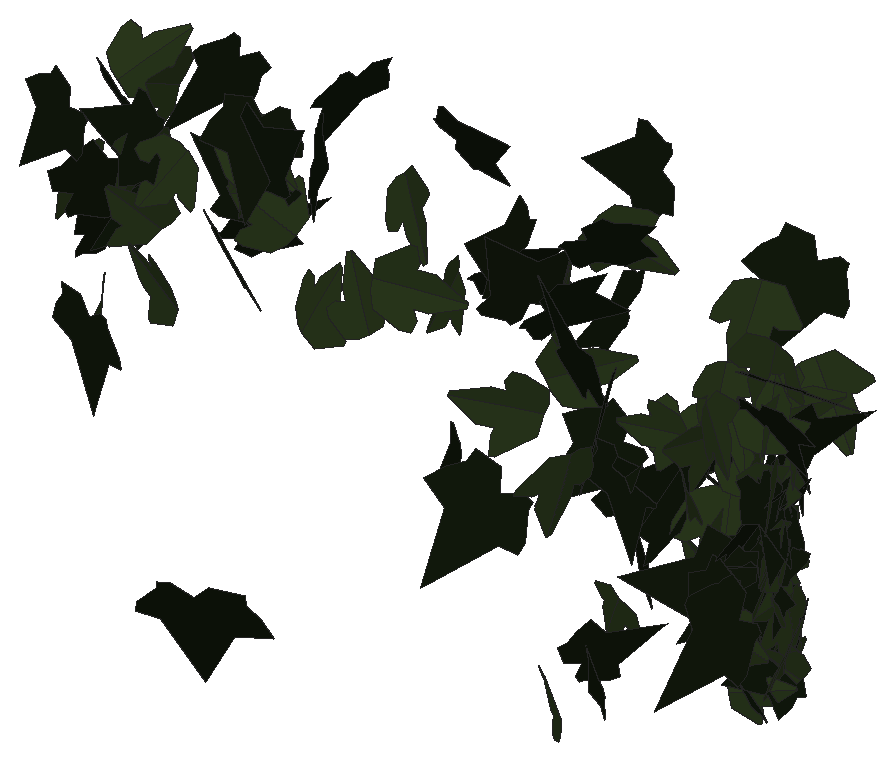
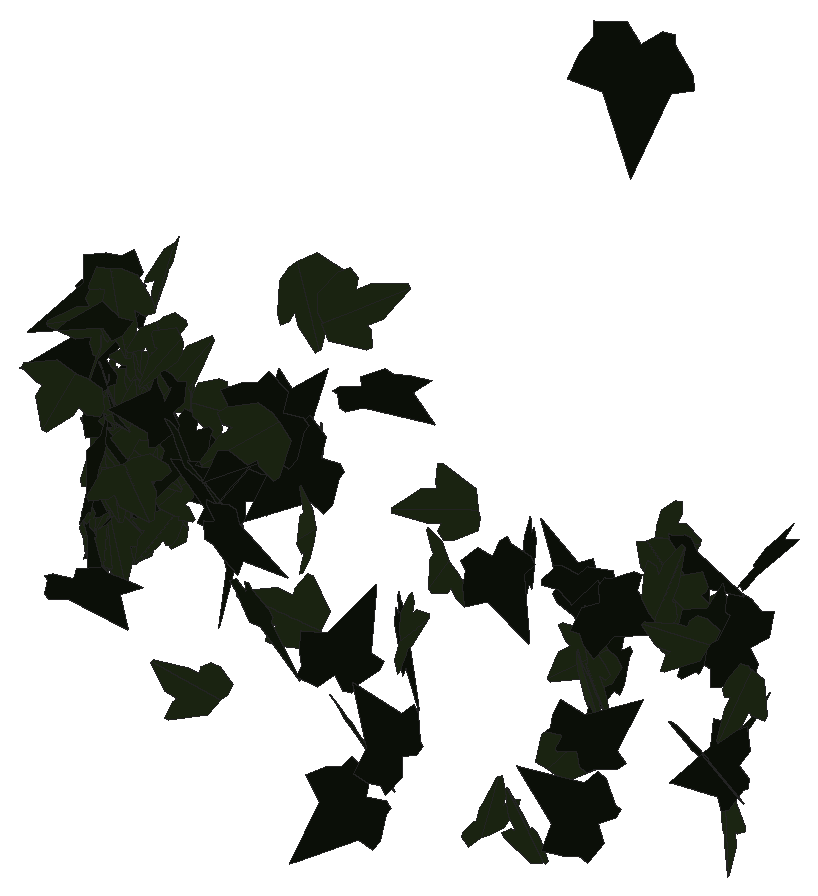
# SketchUp Ruby script. Lengths in inches.
U = 1.inch
M = Sketchup.active_model
def pt(a) = Geom::Point3d.new(a.map { |v| v * U })
def face(e, loops, mat)
  f = e.add_face(loops[0].map { |a| pt(a) })
  loops[1..].each { |l| e.add_face(l.map { |a| pt(a) }).erase! }
  f.material = f.back_material = mat if mat
  f
end
# faces: each face lists its corners as indices into pts; further lists are holes
def faces(e, pts, list, mat = nil) = list.each { |f| face(e, (f[0].is_a?(Array) ? f : [f]).map { |l| l.map { |i| pts[i] } }, mat) }
# xy, xz, yz: faces in a plane at the given z, y or x. An outline is a flat list of corners, or four numbers for a rectangle; further outlines are holes
def ring(l) = l.size == 4 ? [[l[0], l[1]], [l[2], l[1]], [l[2], l[3]], [l[0], l[3]]] : l.each_slice(2).to_a
def flat(e, list, mat, &to3) = list.each { |f| face(e, (f[0].is_a?(Array) ? f : [f]).map { |l| ring(l).map { |u, v| to3.(u, v) } }, mat) }
def xy(e, z, list, mat = nil) = flat(e, list, mat) { |x, y| [x, y, z] }
def xz(e, y, list, mat = nil) = flat(e, list, mat) { |x, z| [x, y, z] }
def yz(e, x, list, mat = nil) = flat(e, list, mat) { |y, z| [x, y, z] }
def lines(e, pts, list) = list.each { |a, b| e.add_line(pt(pts[a]), pt(pts[b])) }
# prism: a flat outline (further loops are holes) pulled along v
def prism(e, loops, v, mat = nil)
  f = face(e, loops, mat); d = Geom::Vector3d.new(v.map { |x| x * U })
  f.pushpull(f.normal.samedirection?(d) ? d.length : -d.length)
end
def box(e, o, s, mat = nil) = prism(e, [[o, [o[0] + s[0], o[1], o[2]], [o[0] + s[0], o[1] + s[1], o[2]], [o[0], o[1] + s[1], o[2]]]], [0, 0, s[2]], mat)
def at(x, y, z, deg = 0) = Geom::Transformation.translation(pt([x, y, z])) * Geom::Transformation.rotation(ORIGIN, Z_AXIS, deg.degrees)
def axes(o, x, y, z) = Geom::Transformation.new([*x, 0, *y, 0, *z, 0, *pt(o).to_a, 1])
def part(name) = M.definitions.add(name)
# library, detail: a bought-in or finely detailed component or shape, given as its bounding box
def library(name, o, s) = part(name).tap { |d| box(d.entities, o, s) }
def detail(e, o, s) = box(e.add_group.entities, o, s)
def put(e, d, t, mat = nil) = e.add_instance(d, t).tap { |i| i.material = mat if mat }
def group(e, t, mat = nil) = e.add_group.tap { |g| g.transformation = t; g.material = mat if mat }.entities
root = M.entities
M.materials.add("efeu1").color = [18, 25, 13]
M.materials.add("efeu2").color = [43, 57, 29]
c1 = part("ivyleaf_9")
p = [[1.54,2.16,1.25],[1.36,2.04,1.19],[-0.21,0.99,0.68],[-0.71,1.11,0.82],[-0.85,0.86,0.67],[-0.8,0.17,0.21],
  [-0.9,-0.01,0.1],[-0.67,-0.16,-0.02],[-0.08,-0.08,-0.05],[-0.03,-0.6,-0.4],[0.65,-0.88,-0.66],[0.83,-0.6,-0.49],
  [1.29,-0.42,-0.43],[1.8125,-0.07,-0.26],[1.21,0.44,0.15]]
faces(c1.entities,p,[[0,1,2,3,4,5,6,7,8,9,10,11,12,13,14]],"efeu1")
c2 = part("ivyleaf_10")
p = [[0,0.5,-0.03],[-0.0625,2.02,-0.43],[-0.19,2.01,-0.46],[-0.54,1.05,-0.29],[-0.52,0.625,-0.18],[-0.83,0.76,-0.28],
  [-1.16,0.64,-0.33],[-1.15,0.33,-0.24],[-0.77,-0.39,0.02],[-0.3,-0.51,0.16],[0.04,-0.48,0.23],[-0.02,2.01,-0.4375],
  [-0.06,2.01,-0.43],[0.04,-0.49,0.23],[0.67,-0.49,0.14],[1.38,0.36,-0.2],[1.375,0.51,-0.24],[0.81,0.65,-0.19],
  [0.62,0.59,-0.15],[0.6,1.09,-0.28],[0.5,1.23,-0.31]]
faces(c2.entities,p,[[0,1,2,3,4,5,6,7,8,9,10],[11,12,0,13,14,15,16,17,18,19,20]],"efeu2")
put(root,c1,axes([559.65,131.34,166.89],[0.18867,0.32237,0.85556],[0.48265,0.70682,-0.37276],[-0.7765,0.51767,-0.02382]))
put(root,c2,axes([559.94,130.49,169.13],[-0.11425,-0.61907,-0.70388],[0.13568,0.6907,-0.6295],[0.92751,-0.1773,0.00538]))
put(root,c2,axes([560.29,130.93,165.03],[0.24542,-0.7584,-0.53558],[-0.16784,0.50861,-0.79712],[0.91315,0.29731,-0.00257]))
put(root,c1,axes([560.9,132.3,167.92],[-0.8896,0.2827,0.00809],[-0.00891,-0.00134,-0.93343],[-0.28267,-0.88963,0.00397]))
put(root,c2,axes([560.07,132.65,171.47],[0.44933,0.18966,-0.7966],[0.58947,0.55578,0.46483],[0.56838,-0.72634,0.14767]))
put(root,c1,axes([560.82,128.91,172.12],[-0.18955,-0.63647,0.63104],[-0.14198,-0.61553,-0.66348],[0.88496,-0.23508,0.02872]))
put(root,c1,axes([560.35,131.88,170.99],[0.35346,-0.64871,0.71095],[0.38408,-0.59938,-0.73786],[0.88247,0.5207,0.03638]))
put(root,c1,axes([560.98,129.21,169.51],[0.27149,0.13056,0.96082],[0.8802,0.38541,-0.30108],[-0.4068,0.92106,-0.01021]))
put(root,c1,axes([561.58,128.91,165.9],[0.21848,-0.9221,0.46101],[0.10195,-0.44961,-0.94763],[1.02587,0.24107,-0.004]))
put(root,c2,axes([561.99,132.11,171.84],[-0.05342,-0.47538,-0.88061],[-0.01757,-0.88128,0.47681],[-1.00058,0.04085,0.03864]))
put(root,c2,axes([562.44,130.49,170.96],[0.05578,-0.79808,0.65077],[0.08026,-0.64637,-0.79956],[1.02664,0.09389,0.02715]))
put(root,c1,axes([563.24,129.375,171.79],[-0.4545,-0.08174,-0.8077],[-0.77073,-0.24731,0.45873],[-0.255,0.89318,0.0531]))
put(root,c1,axes([561.96,135.13,165.86],[0.54216,0.73882,-0.28624],[0.16688,0.23258,0.9164],[0.77456,-0.56726,0.00292]))
put(root,c1,axes([563.07,134.42,167.63],[0.21088,0.02513,0.89081],[-0.88414,0.12062,0.2059],[-0.11169,-0.90745,0.05204]))
put(root,c1,axes([562.83,133.65,172.23],[-0.087,0.09537,-0.95392],[0.20828,-0.93308,-0.11228],[-0.93578,-0.21655,0.0637]))
put(root,c2,axes([563.09,129.71,169.09],[-0.50207,-0.41287,-0.63439],[-0.466,-0.43128,0.64949],[-0.59646,0.68449,0.02657]))
put(root,c2,axes([563.66,134.52,167.09],[0.28232,0.65238,0.63256],[-0.2484,-0.58175,0.71084],[0.87409,-0.37604,-0.0023]))
put(root,c2,axes([563.78,133.26,169.99],[0.73206,-0.45223,-0.41717],[-0.35019,0.22685,-0.86044],[0.50588,0.81147,0.00805]))
put(root,c2,axes([563.67,133.45,169.76],[0.43367,-0.85625,0.09704],[0.04244,-0.08728,-0.95981],[0.86068,0.43574,-0.00157]))
put(root,c2,axes([563.35,133.24,170.18],[0.48471,0.28103,0.77164],[0.66689,0.38819,-0.56029],[-0.47924,0.82443,0.00078]))
put(root,c2,axes([564.25,129.25,171.53],[0.80622,-0.12206,-0.46029],[-0.45675,0.05783,-0.81535],[0.13472,0.92656,-0.00975]))
put(root,c2,axes([564.23,135.14,164.16],[0.8248,-0.33355,-0.39557],[0.37582,-0.12546,0.88941],[-0.35566,-0.90611,0.02247]))
put(root,c1,axes([564.52,130.74,168.7],[0.81404,-0.21703,-0.46569],[-0.44967,0.12109,-0.84248],[0.24852,0.92998,0.00102]))
put(root,c1,axes([564.89,132.12,171.76],[-0.64568,-0.59114,-0.3949],[0.29202,0.26585,-0.87541],[0.64816,-0.70865,0.00101]))
put(root,c2,axes([565.69,135.49,164.54],[0.07983,0.92735,-0.03059],[-0.02138,0.03253,0.93047],[0.92761,-0.07906,0.02407]))
put(root,c1,axes([565.12,131.74,170.72],[-0.1527,0.13015,0.90461],[0.60858,-0.66976,0.19909],[0.68183,0.62695,0.02489]))
put(root,c2,axes([566.63,125.84,169.72],[-0.23736,0.21284,-0.91602],[-0.75913,0.51427,0.3162],[0.55508,0.79433,0.04073]))
put(root,c1,axes([566.46,134.2,172.65],[-0.16332,0.75727,-0.51997],[0.10249,-0.5098,-0.77466],[-0.91287,-0.19272,0.00606]))
put(root,c1,axes([566.03,139.17,168.47],[0.8459,0.03552,-0.51662],[0.51108,0.10211,0.84384],[0.08341,-0.98591,0.06879]))
put(root,c1,axes([567.34,131.38,171.78],[0.10867,0.00701,-0.96456],[-0.86553,0.42917,-0.09439],[0.42578,0.87063,0.0543]))
put(root,c1,axes([568.25,138.13,165.75],[0.68522,0.61936,0.36595],[0.26369,0.25399,-0.92359],[-0.66933,0.73413,0.01079]))
put(root,c1,axes([569.66,136.9,167.21],[-0.52986,0.61283,0.52621],[-0.33329,0.40739,-0.81004],[-0.73579,-0.62585,-0.01202]))
put(root,c2,axes([569.31,132.79,170.84],[0.6838,-0.17805,0.68953],[0.67865,-0.1268,-0.70575],[0.21584,0.96278,0.03457]))
put(root,c2,axes([570.63,133.25,168.27],[-0.00963,0.24464,-0.92655],[0.05628,-0.92485,-0.24478],[-0.95665,-0.05687,-0.00507]))
put(root,c1,axes([571.75,135,167.43],[0.43111,0.27712,0.8202],[-0.73806,-0.36131,0.51001],[0.45254,-0.85326,0.05042]))
put(root,c2,axes([571.6875,129.2,170.39],[0.09174,0.07386,1.0205],[0.80474,0.62754,-0.11776],[-0.63187,0.80995,-0.00182]))
put(root,c1,axes([574.2,128.92,165.61],[-0.00185,0.06279,-1.0646],[-1.05613,0.1476,0.01055],[0.14796,1.05432,0.06193]))
put(root,c1,axes([575,136.47,171.87],[-0.31696,-0.10223,-0.93548],[-0.87148,-0.3406,0.3325],[-0.3551,0.92713,0.01899]))
put(root,c1,axes([575.3,134.64,168.54],[-0.72697,0.66362,0.05925],[-0.04789,0.03543,-0.98429],[-0.66453,-0.72852,0.00611]))
put(root,c2,axes([575.27,131.88,169.51],[0.2964,-0.3148,0.91613],[-0.61495,0.67911,0.43231],[-0.74849,-0.68261,0.00761]))
put(root,c2,axes([574.71,132.79,167.07],[-0.33379,-0.27157,0.93693],[0.69855,0.62466,0.42992],[-0.6809,0.77399,-0.01823]))
put(root,c1,axes([576.3,130.1875,170.83],[0.52629,0.68671,0.54597],[0.34991,0.41953,-0.86498],[-0.80449,0.63171,-0.01905]))
put(root,c1,axes([576.83,131.3125,172.64],[0.79517,0.55938,0.31258],[0.25594,0.17945,-0.97221],[-0.58746,0.83534,-0.00047]))
put(root,c2,axes([576.72,134.84,164.86],[0.53459,0.25007,-0.79473],[0.68146,0.412,0.58804],[0.47932,-0.86466,0.05035]))
put(root,c2,axes([576.78,132.17,172.51],[-0.59931,-0.20053,-0.82563],[0.77443,0.28666,-0.63177],[0.34948,-0.97912,-0.01588]))
put(root,c1,axes([578.74,128.64,170.16],[0.37656,-0.53585,0.84186],[-0.4675,0.70023,0.65481],[-0.88165,-0.60017,0.01234]))
put(root,c1,axes([578.78,138.375,169.5],[-0.84373,-0.64162,-0.07423],[0.06169,0.04151,-1.05997],[0.64295,-0.84597,0.00429]))
put(root,c1,axes([579.7,123.67,169.19],[-0.832,-0.6765,0.1782],[-0.12865,-0.12422,-1.07222],[0.68765,-0.84175,0.01501]))
put(root,c2,axes([580.25,124.22,171.73],[-0.24784,-0.18247,-1.01726],[-0.84053,-0.5731,0.30758],[-0.60135,0.87624,-0.01066]))
put(root,c1,axes([580.125,128.39,168.85],[-0.84228,-0.35801,0.2763],[-0.25264,-0.11193,-0.9152],[0.37508,-0.87935,0.004]))
put(root,c1,axes([579.79,128.37,170.4],[-0.47843,0.2548,-0.82492],[0.72483,-0.39387,-0.54203],[-0.46908,-0.86848,0.0038]))
put(root,c2,axes([580.1875,134.18,170.77],[0.63243,0.71801,-0.31985],[-0.22658,-0.22658,-0.95663],[-0.75267,0.67152,0.01922]))
put(root,c1,axes([580.74,128.43,165.86],[0.49352,-0.15456,-0.74391],[-0.70673,0.23232,-0.51712],[0.27897,0.86198,0.00599]))
put(root,c1,axes([580.42,128.24,168.27],[0.18772,-0.91784,0.2521],[0.06357,-0.24429,-0.93675],[0.9497,0.19777,0.01287]))
put(root,c1,axes([580.66,128.25,167.1],[-0.12386,-0.04505,0.94856],[0.8802,0.35359,0.13173],[-0.35642,0.88887,-0.00432]))
put(root,c1,axes([581.52,108.52,173.26],[0.82611,0.77267,-0.61847],[-0.45471,-0.41924,-1.13113],[-0.87907,0.94298,0.00388]))
put(root,c2,axes([581.98,128.3,169.87],[0.06419,-0.01698,-0.80888],[-0.8075,0.04905,-0.06511],[0.05024,0.80994,-0.01302]))
put(root,c1,axes([582.5,128.19,168.06],[-0.83385,0.98017,0.38971],[-0.24907,0.29975,-1.28686],[-1.02497,-0.87024,-0.00432]))
put(root,c1,axes([582.14,128.7,169],[0.77452,0.13114,-0.32505],[-0.34838,0.20134,-0.74889],[-0.03854,0.81548,0.23717]))
put(root,c2,axes([582.66,122.91,171.42],[-0.19533,-1.08173,0.13943],[-0.02031,-0.13802,-1.09921],[1.09049,-0.19634,0.0045]))
put(root,c2,axes([583.02,124.75,166.55],[-0.62436,0.05711,0.37828],[-0.37682,0.03331,-0.62696],[-0.0661,-0.72925,0.00099]))
put(root,c2,axes([582.77,122.32,164.22],[-0.6276,0.50849,0.402],[0.29657,-0.2723,0.80743],[0.57638,0.69379,0.02228]))
put(root,c2,axes([583.58,128.125,166.05],[-0.52864,0.05127,-0.47737],[-0.47453,0.05215,0.5311],[0.07299,0.71037,-0.00454]))
put(root,c2,axes([583.27,128.34,170.15],[-0.09977,-0.23968,-0.99069],[-0.2072,-0.96988,0.25551],[-0.99799,0.22532,0.046]))
put(root,c1,axes([582.9375,123.95,164.64],[-0.00179,-0.19249,0.77784],[0.09287,-0.77265,-0.191],[0.7959,0.08973,0.02404]))
put(root,c2,axes([583.26,128.33,171.33],[-0.00458,0.3102,0.70886],[-0.13444,0.69777,-0.30622],[-0.76199,-0.12498,0.04977]))
put(root,c1,axes([583.02,128.71,169.4375],[0.14429,0.13152,0.77329],[0.52809,0.56508,-0.19465],[-0.57999,0.54724,0.01515]))
put(root,c1,axes([582.86,123.5,165.3125],[0.17182,0.03508,0.80915],[0.73999,0.32938,-0.17142],[-0.32917,0.75878,0.037]))
put(root,c2,axes([583.99,128.78,167.53],[-0.27152,-0.11536,0.65479],[-0.60873,-0.24132,-0.29494],[0.2674,-0.66651,-0.00655]))
put(root,c2,axes([583.52,128.61,172],[0.36041,0.65573,-0.21436],[-0.11075,-0.18372,-0.7482],[-0.68093,0.37695,0.00823]))
put(root,c2,axes([583.37,128.5,165.45],[0.19005,0.53293,0.44857],[0.11562,0.43438,-0.56507],[-0.68692,0.22056,0.029]))
put(root,c2,axes([583.62,128.68,167.45],[0.07222,0.52226,-0.52243],[-0.09608,-0.51382,-0.52694],[-0.73243,0.1189,0.01761]))
put(root,c2,axes([584.03,126.49,169.5],[-0.46902,0.26496,0.34766],[-0.30342,0.16973,-0.53869],[-0.31466,-0.5586,0.00123]))
put(root,c1,axes([583.16,131.95,168.84],[0.27284,-0.07466,-1.03772],[0.97842,-0.34636,0.28217],[-0.35375,-1.01555,-0.01994]))
put(root,c2,axes([583.73,128.45,168.07],[1.11952,0.51087,-0.02154],[-0.02248,-0.00262,-1.23055],[-0.51083,1.11972,0.00695]))
put(root,c2,axes([583.41,127.79,165.2],[-0.00748,0.01722,-0.73226],[0.58619,-0.43895,-0.01631],[-0.43919,-0.58616,-0.0093]))
put(root,c2,axes([584.54,128.65,170.21],[-0.07169,0.06244,0.67636],[-0.66441,0.13488,-0.08288],[-0.14114,-0.66664,0.04659]))
put(root,c2,axes([584.11,128.78,168.92],[0.46004,0.53984,-0.11877],[0.06971,0.09662,0.70921],[0.54834,-0.4652,0.00948]))
put(root,c2,axes([584.06,128.68,170.85],[0.67589,0.26893,0.10796],[0.09917,0.04279,-0.72742],[-0.2723,0.68312,0.00307]))
put(root,c1,axes([585.11,126.88,166.73],[-0.52672,-0.0226,0.88778],[-0.8754,-0.16054,-0.52346],[0.1495,-1.01972,0.06274]))
put(root,c2,axes([585.36,128.08,167.21],[0.00562,0.03633,0.91204],[-0.89783,0.1645,-0.00102],[-0.16441,-0.8971,0.03675]))
put(root,c1,axes([585.45,126.25,166.83],[-0.40153,-0.17588,-0.72276],[-0.6437,-0.32945,0.43778],[-0.37278,0.75833,0.02256]))
put(root,c2,axes([584.9,128.9375,166.65],[0.60026,0.17533,-0.12751],[-0.19101,0.25018,-0.55519],[-0.10254,0.56034,0.28778]))
put(root,c2,axes([584.97,128.75,173],[1.0213,-0.04859,-0.26336],[-0.23218,0.35682,-0.9662],[0.13346,0.99252,0.33446]))
put(root,c1,axes([585.36,128.02,168.47],[-0.67767,0.39309,-0.49562],[-0.43604,0.23592,0.78332],[0.45828,0.80574,0.01243]))
put(root,c2,axes([584.52,131.47,171.08],[0.86408,0.39509,0.51358],[0.4661,0.2157,-0.95012],[-0.45013,0.98177,0.00207]))
put(root,c2,axes([585.18,128.92,168.23],[-0.22117,-0.60709,0.16967],[-0.07041,-0.1549,-0.64599],[0.62641,-0.23176,-0.0127]))
put(root,c1,axes([585.49,127.52,166.69],[0.03461,0.14296,-0.90903],[-0.29489,-0.85998,-0.14647],[-0.87168,0.29661,0.01346]))
put(root,c1,axes([585.38,128.26,165.26],[-0.47318,-0.6625,0.27004],[0.15498,0.22115,0.81412],[-0.69843,0.49791,-0.0023]))
put(root,c2,axes([585.41,128.48,164.45],[-0.72286,-0.18992,0.32912],[-0.31884,-0.08163,-0.74739],[0.20671,-0.79005,-0.0019]))
put(root,c1,axes([585.43,129.07,164.01],[-0.01765,0.29792,0.83183],[-0.09419,0.82662,-0.29805],[-0.87854,-0.09461,0.01525]))
put(root,c2,axes([585.24,128.6,169.64],[-0.5932,-0.39277,0.05138],[-0.04325,-0.02774,-0.71145],[0.39375,-0.59478,-0.00074]))
put(root,c1,axes([585.48,127.47,168.77],[-0.33271,0.8503,-0.25234],[0.09338,-0.23443,-0.91307],[-0.88202,-0.34556,-0.00148]))
put(root,c2,axes([585.27,128.93,166.96],[-0.42565,-0.51887,0.05615],[-0.03561,-0.04341,-0.67112],[0.52069,-0.42713,0.00001]))
put(root,c1,axes([585.3,127.32,163.73],[0.53043,-0.7412,0.21735],[-0.12586,0.1772,0.91145],[-0.76209,-0.54516,0.00075]))
put(root,c1,axes([585.6,128.71,168.75],[-0.33887,0.65408,-0.22103],[0.0956,-0.1994,-0.73662],[-0.68377,-0.35204,0.00655]))
put(root,c2,axes([585.4,127.93,166.33],[0.29784,-0.63068,-0.0765],[-0.031,0.06996,-0.69747],[0.63454,0.29945,0.00183]))
put(root,c2,axes([585.58,127.88,166.26],[-0.59093,0.22281,0.24019],[-0.22707,0.07852,-0.63151],[-0.23616,-0.63303,0.0062]))
put(root,c2,axes([585.38,125.82,172.61],[-0.24204,0.87049,0.13535],[-0.05496,0.12517,-0.90331],[-0.87923,-0.24746,0.01921]))
put(root,c2,axes([585.375,128.72,169.1],[0.58524,-0.27707,0.00806],[-0.00721,0.0036,0.64752],[-0.2771,-0.58529,0.00017]))
put(root,c2,axes([585.4,128.89,163.85],[-0.12986,-0.5381,-0.32264],[0.02262,-0.33328,0.54674],[-0.62701,0.09942,0.08655]))
put(root,c1,axes([585.69,127.86,167.23],[-0.71643,0.11059,0.31823],[0.31451,-0.04851,0.72492],[0.12076,0.78243,-0.00004]))
put(root,c2,axes([585.5625,128.45,171.78],[0.07757,-0.4633,0.43277],[0.17578,-0.40319,-0.46314],[0.60913,0.17535,0.07854]))
put(root,c1,axes([585.02,128.3,172.61],[1.03631,-0.04901,0.25065],[0.25171,0.37344,-0.96766],[-0.04326,0.99866,0.37415]))
put(root,c2,axes([585.47,128.53,169.61],[-0.08529,0.4534,-0.65689],[0.11664,-0.64646,-0.46134],[-0.7896,-0.14447,0.0028]))
put(root,c2,axes([585.57,127.89,171.21],[0.50044,0.65119,-0.19633],[0.12095,0.15466,0.82127],[0.6693,-0.51484,-0.00161]))
put(root,c1,axes([586.1875,125.75,166.67],[-1.16114,0.06157,-0.11536],[0.11496,-0.01056,-1.16276],[-0.06231,-1.16681,0.00444]))
put(root,c2,axes([585.85,127.82,167.77],[0.05381,-0.45281,-0.59538],[-0.05667,0.59274,-0.45592],[0.74586,0.0777,0.00831]))
put(root,c2,axes([585.6,128.875,170.6875],[-0.23216,0.47777,-0.36483],[0.13579,-0.3393,-0.53075],[-0.58559,-0.26809,0.02156]))
put(root,c2,axes([586.11,128.25,163.98],[-0.40316,-0.19238,-0.49746],[-0.4399,-0.23269,0.44649],[-0.3016,0.59654,0.01374]))
put(root,c2,axes([585.85,127.92,167.8125],[0.00554,0.4501,-0.54186],[0.00316,0.54185,0.45013],[0.70441,-0.00597,0.00224]))
put(root,c1,axes([585.5,127.71,169.68],[0.33464,-0.67625,-0.22913],[-0.10329,0.20453,-0.75452],[0.7065,0.35022,-0.00178]))
put(root,c2,axes([585.3125,127.19,163.65],[0.11207,-0.01917,-0.71522],[0.70152,0.14524,0.10603],[0.14063,-0.70923,0.04105]))
put(root,c2,axes([585.76,128.5,165.67],[0.10611,-0.93759,-0.18219],[0.22109,0.20245,-0.91305],[0.92918,0.0589,0.23806]))
put(root,c2,axes([585.9375,128.0625,164.17],[0.11679,-0.60786,-0.26917],[-0.04809,0.26485,-0.61897],[0.66304,0.12627,0.00252]))
put(root,c1,axes([585.47,128.8,170.375],[0.33306,0.255,0.85863],[0.62962,0.58491,-0.41794],[-0.63707,0.71138,0.03585]))
put(root,c1,axes([585.89,128.28,164.11],[0.16505,-0.5373,-0.56239],[0.16202,-0.53855,0.56208],[-0.76074,-0.23127,-0.0023]))
put(root,c2,axes([585.43,128.53,171.74],[-0.00774,-0.0042,-0.92703],[0.66818,0.6426,-0.00849],[0.64261,-0.66822,-0.00234]))
put(root,c2,axes([585.78,128.31,166.16],[-0.03888,0.05618,0.70686],[0.23921,-0.66538,0.06604],[0.66752,0.24172,0.01751]))
put(root,c1,axes([585.76,127.49,172.13],[0.85823,0.2173,-0.28923],[-0.28306,-0.06034,-0.88525],[-0.22528,0.90364,0.01044]))
put(root,c2,axes([585.91,128.02,163.91],[0.30777,-0.62384,0.42316],[-0.16147,0.39191,0.6952],[-0.73632,-0.3467,0.02442]))
put(root,c2,axes([585.4,126.65,165.61],[-0.0607,-0.04285,-0.78291],[0.69025,-0.37543,-0.03297],[-0.37195,-0.6897,0.06659]))
put(root,c2,axes([585.95,128.03,168.29],[0.16113,-0.59143,0.42701],[0.13028,-0.40694,-0.61279],[0.71774,0.20664,0.01537]))
put(root,c2,axes([585.71,127.82,167.34],[0.51285,-0.57735,-0.29413],[0.19476,-0.22041,0.77224],[-0.618,-0.54859,-0.00072]))
put(root,c2,axes([585.95,128.05,167.78],[0.66274,-0.62094,0.08992],[0.06564,-0.06145,-0.90818],[0.62398,0.66598,0.00004]))
put(root,c1,axes([585.72,128.22,168.86],[0.047,-0.77097,0.34176],[0.01818,-0.34128,-0.7724],[0.84312,0.05034,-0.0024]))
